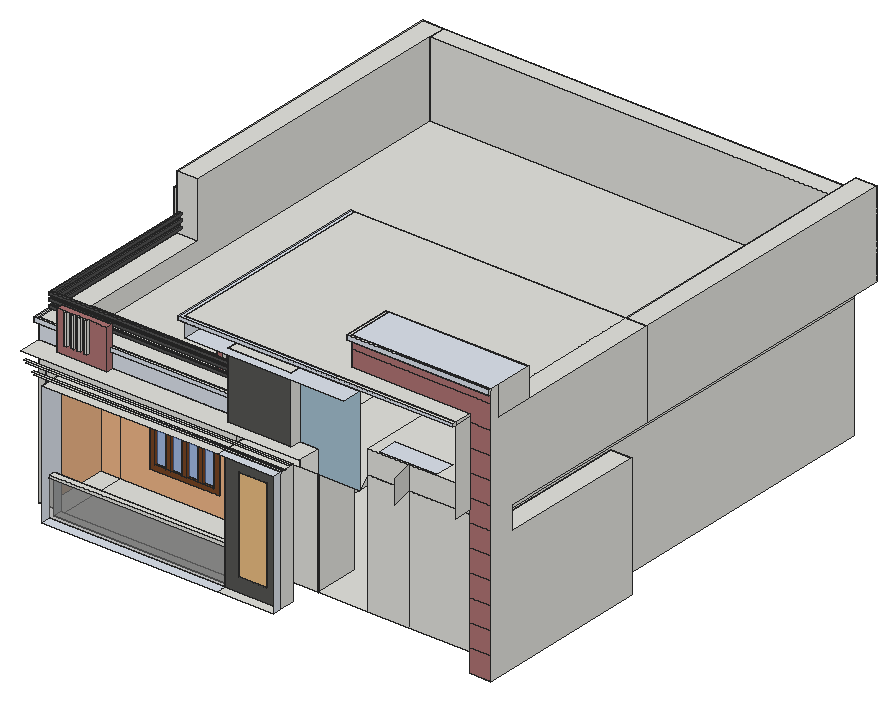
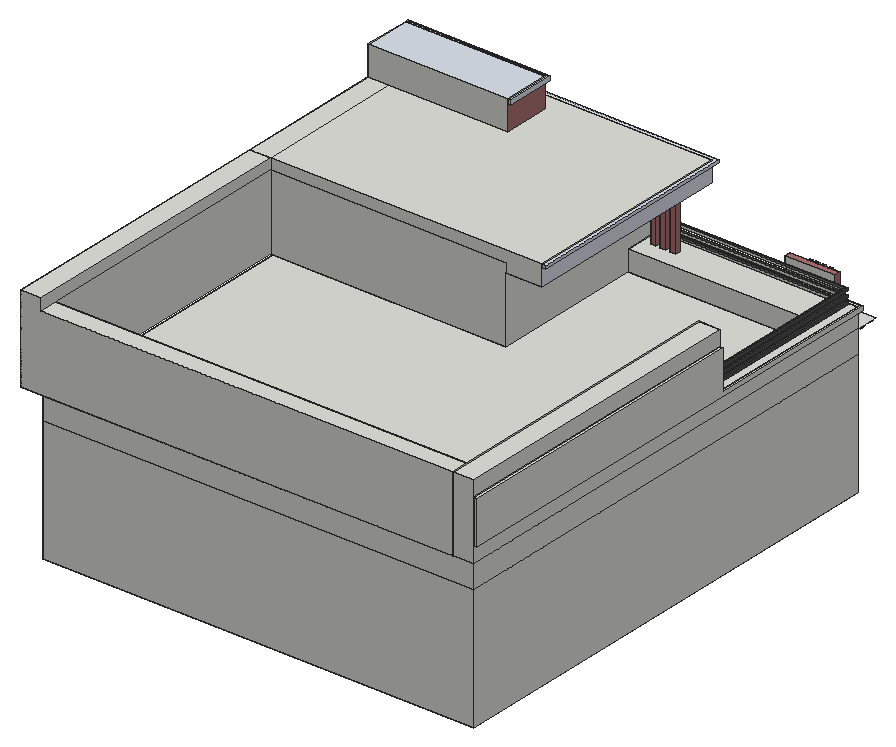
# SketchUp Ruby script. Lengths in inches.
U = 1.inch
M = Sketchup.active_model
def pt(a) = Geom::Point3d.new(a.map { |v| v * U })
def face(e, loops, mat)
  f = e.add_face(loops[0].map { |a| pt(a) })
  loops[1..].each { |l| e.add_face(l.map { |a| pt(a) }).erase! }
  f.material = f.back_material = mat if mat
  f
end
# faces: each face lists its corners as indices into pts; further lists are holes
def faces(e, pts, list, mat = nil) = list.each { |f| face(e, (f[0].is_a?(Array) ? f : [f]).map { |l| l.map { |i| pts[i] } }, mat) }
# xy, xz, yz: faces in a plane at the given z, y or x. An outline is a flat list of corners, or four numbers for a rectangle; further outlines are holes
def ring(l) = l.size == 4 ? [[l[0], l[1]], [l[2], l[1]], [l[2], l[3]], [l[0], l[3]]] : l.each_slice(2).to_a
def flat(e, list, mat, &to3) = list.each { |f| face(e, (f[0].is_a?(Array) ? f : [f]).map { |l| ring(l).map { |u, v| to3.(u, v) } }, mat) }
def xy(e, z, list, mat = nil) = flat(e, list, mat) { |x, y| [x, y, z] }
def xz(e, y, list, mat = nil) = flat(e, list, mat) { |x, z| [x, y, z] }
def yz(e, x, list, mat = nil) = flat(e, list, mat) { |y, z| [x, y, z] }
def lines(e, pts, list) = list.each { |a, b| e.add_line(pt(pts[a]), pt(pts[b])) }
# prism: a flat outline (further loops are holes) pulled along v
def prism(e, loops, v, mat = nil)
  f = face(e, loops, mat); d = Geom::Vector3d.new(v.map { |x| x * U })
  f.pushpull(f.normal.samedirection?(d) ? d.length : -d.length)
end
def box(e, o, s, mat = nil) = prism(e, [[o, [o[0] + s[0], o[1], o[2]], [o[0] + s[0], o[1] + s[1], o[2]], [o[0], o[1] + s[1], o[2]]]], [0, 0, s[2]], mat)
def at(x, y, z, deg = 0) = Geom::Transformation.translation(pt([x, y, z])) * Geom::Transformation.rotation(ORIGIN, Z_AXIS, deg.degrees)
def axes(o, x, y, z) = Geom::Transformation.new([*x, 0, *y, 0, *z, 0, *pt(o).to_a, 1])
def part(name) = M.definitions.add(name)
# library, detail: a bought-in or finely detailed component or shape, given as its bounding box
def library(name, o, s) = part(name).tap { |d| box(d.entities, o, s) }
def detail(e, o, s) = box(e.add_group.entities, o, s)
def put(e, d, t, mat = nil) = e.add_instance(d, t).tap { |i| i.material = mat if mat }
def group(e, t, mat = nil) = e.add_group.tap { |g| g.transformation = t; g.material = mat if mat }.entities
root = M.entities
M.materials.add("Generic").color = [175, 116, 116]
M.materials.add("Generic\#2").color = [164, 192, 208]
M.materials.add("Generic\#3").color = [219, 225, 235]
M.materials.add("Generic\#4").color = [240, 183, 136]
M.materials.add("[0135_DarkGray]").color = [81, 81, 81]
M.materials.add("[Granite Light Gray]").color = [86, 86, 83]
M.materials.add("[Translucent Glass Blue]").color = [100, 149, 237]
M.materials["[Translucent Glass Blue]"].alpha = 0.5
M.materials.add("[Translucent Glass Gray]").color = [128, 128, 128]
M.materials["[Translucent Glass Gray]"].alpha = 0.5
M.materials.add("[Wood Veneer 01]").color = [120, 70, 37]
c1 = library("Group\#6",[0,0,0],[40.87,87.01,0.59])
xy(root,142.6875,[[195.4375,77.59,250.5625,86.22],[195.4375,86.22,250.5625,100.72],[195.4375,91.75,195.4375,100.72,24.3125,100.72,24.3125,91.92],[425.125,98.72,445.5,270.09],[3.0625,100.72,3.0625,568.65,423.0625,568.65,423.0625,175.9,304.375,175.9,304.375,124.65,256.02,124.65,256.02,168.65,9.0625,168.65,9.0625,100.72],
  [9.0625,100.72,28.3125,168.65],[28.3125,100.72,28.3125,168.65,256.02,168.65,256.02,124.65,195.4375,124.65,195.4375,100.72],[304.375,124.65,423.0625,175.9]])
xy(root,142.6875,[[24.3125,77.59,195.4375,77.59,195.4375,86.22,24.3125,86.39]],"Generic\#3")
xy(root,148.78,[[149.02,168.65,188.52,344.59]])
xy(root,156.78,[[209.53,86.22,236.47,90.65]])
xy(root,160.95,[[56.18,168.65,124.43,344.59]])
xy(root,178,[[195.4375,86.22,24.3125,86.39,24.3125,91.92,195.4375,91.75]])
xy(root,181,[[195.4375,86.22,195.4375,91.75,24.3125,91.92,24.3125,86.39]])
xy(root,227.7,[[56.18,168.65,124.43,344.59]])
xy(root,229.03,[[149.02,168.65,188.52,344.59]])
xy(root,248.59,[[209.53,86.22,236.47,90.65]])
xy(root,262.6875,[[24.3125,77.59,195.4375,100.72],[195.4375,86.22,195.4375,124.65,257,124.65,257,100.72,250.5625,100.72,250.5625,86.22],[3.0625,100.72,3.0625,568.65,423.0625,568.65,423.0625,175.9,304.375,175.9,304.375,124.65,316,100.72,257,100.72,257,124.65,256.02,124.65,256.02,168.65,9.0625,168.65,9.0625,100.72],[9.0625,100.72,28.3125,168.65],[28.3125,100.72,28.3125,168.65,256.02,168.65,256.02,124.65,195.4375,124.65,195.4375,100.72],
  [304.375,124.65,423.0625,175.9],[425.125,124.65,445.5,270.09]])
xy(root,262.6875,[[195.4375,77.59,250.5625,86.22]],"Generic\#3")
xy(root,270.625,[[17.8125,75.97,259.625,77.59]])
xy(root,272.67,[[15.77,75.97,261.67,77.59]])
xy(root,278.3,[[10.13,75.97,267.3,77.59]])
xy(root,280.38,[[8.06,75.97,269.38,77.59]])
xy(root,285.375,[[[3.0625,77.59,274.375,77.59,274.375,100.72,257,100.72,257,90.65,195.4375,90.65,195.4375,100.72,3.0625,100.72],[25.83,93.51,74.7,99.88]],[195.4375,90.65,257,100.72],[3.0625,100.72,3.0625,568.65,23.25,568.65,23.25,139.72,195.4375,139.72,195.4375,100.72],[195.4375,100.72,257,124.65],[423.0625,100.72,425.125,124.65],
  [195.4375,124.65,257,289.03],[304.375,124.65,423.0625,289.03],[423.0625,124.65,425.125,289.03],[425.125,124.65,445.5,289.03],[23.25,139.72,195.4375,139.72,195.4375,289.03,423.0625,289.03,423.0625,551.28,23.25,551.28],
  [425.125,289.03,425.125,551.28,423.0625,551.28,423.0625,568.65,445.5,568.65,445.5,289.03],[23.25,551.28,423.0625,568.65]])
xy(root,294.7,[[34.08,91.94,37.39,93.51],[40.58,91.94,43.89,93.51],[47.08,91.94,50.39,93.51],[53.58,91.94,56.89,93.51]])
xy(root,301.3125,[[0,97.65,0,568.65,3.0625,568.65,3.0625,100.72,195.4375,100.72,195.4375,97.65]])
xy(root,305.0625,[[0,97.65,195.4375,97.65,195.4375,100.72,3.0625,100.72,3.0625,268.56,0,268.56],[[3.0625,100.72,195.4375,100.72,195.4375,139.72,23.25,139.72,23.25,268.56,3.0625,268.56],[161.83,118.97,167.81,123.29],[171.57,118.97,177.49,123.29],[181.31,118.97,186.72,123.29]]])
xy(root,317.5625,[[350.4375,81.53,406.3,100.72]],"Generic\#3")
xy(root,324.14,[[34.08,91.94,37.39,93.51],[40.58,91.94,43.89,93.51],[47.08,91.94,50.39,93.51],[53.58,91.94,56.89,93.51]])
xy(root,324.14,[[25.83,93.51,74.7,99.88]],"Generic")
xy(root,343.9375,[[0,268.56,3.0625,568.65]])
xy(root,349.9375,[[195.4375,90.65,257,100.72],[160.125,100.72,195.4375,289.03]])
xy(root,349.9375,[[160.125,81.53,160.125,100.72,195.4375,100.72,195.4375,90.65,257,90.65,257,100.72,316,100.72,316,81.53]],"Generic\#3")
xy(root,355.6875,[[161.83,118.97,167.81,123.29],[171.57,118.97,177.49,123.29],[181.31,118.97,186.72,123.29]])
xy(root,358.8125,[[3.0625,268.56,23.25,568.65],[23.25,551.28,425.125,568.65]])
xy(root,366.8125,[[156.8125,77.97,156.8125,289.03,160.125,289.03,160.125,81.53,193.5,81.53,193.5,77.97],[193.5,77.97,425.125,81.53]])
xy(root,369.6875,[[309.3125,77.97,425.125,81.53],[160.125,81.53,425.125,81.53,425.125,98.72,309.3125,98.72,309.3125,144.28,425.125,144.28,425.125,289.03,160.125,289.03],[425.125,144.28,445.5,289.03],[425.125,289.03,445.5,568.65]])
xy(root,369.6875,[[156.8125,77.97,309.3125,77.97,309.3125,81.53,160.125,81.53,160.125,289.03,156.8125,289.03]],"Generic\#3")
xy(root,393.625,[[306.625,96.53,306.625,144.28,309.3125,144.28,309.3125,98.72,445.5,98.72,445.5,96.53]])
xy(root,398.0625,[[306.625,96.53,445.5,96.53,445.5,98.72,309.3125,98.72,309.3125,144.28,306.625,144.28]])
xy(root,398.0625,[[309.3125,98.72,445.5,144.28]],"Generic\#3")
xz(root,77.97,[[156.8125,366.8125,425.125,369.6875]],"Generic\#3")
xz(root,81.53,[[160.125,366.8125,193.5,369.6875],[193.5,366.8125,425.125,369.6875]])
xz(root,86.22,[[[195.4375,142.6875,250.5625,262.6875],[209.53,156.78,236.47,248.59]]],"[Granite Light Gray]")
xz(root,90.65,[[209.53,156.78,236.47,248.59]])
xz(root,90.65,[[195.4375,285.375,257,349.9375]],"[Granite Light Gray]")
xz(root,91.94,[[34.08,294.7,37.39,324.14],[40.58,294.7,43.89,324.14],[47.08,294.7,50.39,324.14],[53.58,294.7,56.89,324.14]])
xz(root,93.51,[[34.08,294.7,37.39,324.14],[40.58,294.7,43.89,324.14],[47.08,294.7,50.39,324.14],[53.58,294.7,56.89,324.14]])
xz(root,93.51,[[25.83,285.375,74.7,285.375,74.7,324.14,56.89,324.14,56.89,294.7,53.58,294.7,53.58,324.14,50.39,324.14,50.39,294.7,47.08,294.7,47.08,324.14,43.89,324.14,43.89,294.7,40.58,294.7,40.58,324.14,37.39,324.14,37.39,294.7,34.08,294.7,34.08,324.14,25.83,324.14]],"Generic")
xz(root,96.53,[[306.625,393.625,445.5,398.0625]],"Generic\#3")
xz(root,97.65,[[0,301.3125,195.4375,305.0625]],"Generic\#3")
xz(root,98.72,[[309.3125,393.625,445.5,398.0625]])
xz(root,98.72,[[425.125,142.6875,445.5,164.62],[425.125,164.62,445.5,186.55],[425.125,186.55,445.5,208.48],[425.125,208.48,445.5,230.41],[425.125,230.41,445.5,252.35],
  [425.125,252.35,445.5,274.28],[425.125,274.28,445.5,296.21],[425.125,296.21,445.5,318.14],[425.125,318.14,445.5,340.07],[425.125,340.07,445.5,362],
  [425.125,362,445.5,362,445.5,385.625,309.3125,385.625,309.3125,369.6875,425.125,369.6875],[309.3125,385.625,445.5,393.625]],"Generic")
xz(root,99.88,[[25.83,285.375,74.7,324.14]])
xz(root,100.72,[[9.0625,142.6875,24.3125,262.6875],[3.0625,262.6875,195.4375,285.375],[257,262.6875,274.375,285.375],[423.0625,262.6875,425.125,285.375],[195.4375,285.375,257,349.9375],
  [3.0625,301.3125,195.4375,305.0625]])
xz(root,100.72,[[274.375,262.6875,316,262.6875,316,349.9375,257,349.9375,257,285.375,274.375,285.375]],"Generic\#2")
xz(root,100.72,[[3.0625,285.375,195.4375,301.3125]],"Generic\#3")
xz(root,118.97,[[161.83,305.0625,167.81,355.6875],[171.57,305.0625,177.49,355.6875],[181.31,305.0625,186.72,355.6875]],"Generic")
xz(root,123.29,[[161.83,305.0625,167.81,355.6875],[171.57,305.0625,177.49,355.6875],[181.31,305.0625,186.72,355.6875]],"Generic")
xz(root,124.65,[[195.4375,142.6875,256.02,262.6875],[256.02,142.6875,257,262.6875],[304.375,142.6875,344.25,262.6875],[344.25,142.6875,423.0625,262.6875],[195.4375,262.6875,257,285.375],
  [304.375,262.6875,344.25,285.375],[344.25,262.6875,425.125,285.375],[425.125,262.6875,445.5,285.375]])
xz(root,139.72,[[23.25,285.375,195.4375,305.0625]])
xz(root,144.28,[[309.3125,369.6875,445.5,398.0625],[306.625,393.625,309.3125,398.0625]])
xz(root,168.65,[[9.0625,142.6875,28.3125,262.6875],[[28.3125,142.6875,256.02,262.6875],[56.18,160.95,124.43,227.7],[149.02,148.78,188.52,229.03]]],"Generic\#4")
xz(root,175.9,[[304.375,142.6875,423.0625,262.6875]])
xz(root,268.56,[[0,305.0625,3.0625,343.9375],[3.0625,305.0625,23.25,358.8125]])
xz(root,270.09,[[425.125,142.6875,445.5,262.6875]])
xz(root,270.23,[[7.9,321.65,5.61,321.7,5.59,324.14,7.875,324.09]])
xz(root,271.04,[[7.9,316.02,5.61,316.07,5.59,318.52,7.875,318.47]])
xz(root,273.16,[[7.9,309.96,5.61,310.01,5.59,312.46,7.875,312.4]])
xz(root,289.03,[[195.4375,285.375,195.4375,358.5625,257,358.5625,257,358.8125,425.125,358.8125,425.125,285.375],[425.125,285.375,445.5,369.6875],[160.125,349.9375,160.125,369.6875,425.125,369.6875,425.125,358.8125,257,358.8125,257,358.5625,195.4375,358.5625,195.4375,349.9375],[156.8125,366.8125,160.125,369.6875]])
xz(root,344.59,[[149.02,148.78,188.52,229.03],[56.18,160.95,124.43,227.7]])
xz(root,551.28,[[23.25,285.375,425.125,358.8125]])
xz(root,568.65,[[3.0625,142.6875,423.0625,262.6875],[3.0625,262.6875,423.0625,285.375],[3.0625,285.375,23.25,358.8125],[23.25,285.375,23.25,358.8125,425.125,358.8125,425.125,369.6875,445.5,369.6875,445.5,285.375],[0,301.3125,3.0625,343.9375]])
yz(root,0,[[97.65,301.3125,97.65,305.0625,268.56,305.0625,268.56,343.9375,568.65,343.9375,568.65,301.3125]])
yz(root,3.0625,[[100.72,142.6875,568.65,262.6875],[100.72,262.6875,568.65,285.375],[100.72,285.375,568.65,301.3125],[100.72,301.3125,568.65,301.3125,568.65,343.9375,268.56,343.9375,268.56,305.0625,100.72,305.0625],[268.56,343.9375,568.65,358.8125]])
yz(root,9.0625,[[100.72,142.6875,168.65,262.6875]],"Generic\#4")
yz(root,23.25,[[139.72,285.375,551.28,285.375,551.28,358.8125,268.56,358.8125,268.56,305.0625,139.72,305.0625],[551.28,285.375,568.65,358.8125]])
yz(root,24.3125,[[86.39,178,91.92,181]])
yz(root,24.3125,[[77.59,142.6875,86.39,142.6875,86.39,181,91.92,181,91.92,142.6875,100.72,142.6875,100.72,262.6875,77.59,262.6875]],"Generic\#3")
yz(root,25.83,[[93.51,285.375,99.88,324.14]],"Generic")
yz(root,34.08,[[91.94,294.7,93.51,324.14]])
yz(root,37.39,[[91.94,294.7,93.51,324.14]])
yz(root,40.58,[[91.94,294.7,93.51,324.14]])
yz(root,43.89,[[91.94,294.7,93.51,324.14]])
yz(root,47.08,[[91.94,294.7,93.51,324.14]])
yz(root,50.39,[[91.94,294.7,93.51,324.14]])
yz(root,53.58,[[91.94,294.7,93.51,324.14]])
yz(root,56.18,[[168.65,160.95,344.59,227.7]])
yz(root,56.89,[[91.94,294.7,93.51,324.14]])
yz(root,74.7,[[93.51,285.375,99.88,324.14]],"Generic")
yz(root,124.43,[[168.65,160.95,344.59,227.7]])
yz(root,149.02,[[168.65,148.78,344.59,229.03]])
yz(root,156.8125,[[77.97,366.8125,289.03,369.6875]],"Generic\#3")
yz(root,160.125,[[81.53,366.8125,289.03,369.6875]])
yz(root,160.125,[[81.53,349.9375,289.03,366.8125]],"Generic\#3")
yz(root,161.83,[[118.97,305.0625,123.29,355.6875]],"Generic")
yz(root,167.81,[[118.97,305.0625,123.29,355.6875]])
yz(root,171.57,[[118.97,305.0625,123.29,355.6875]],"Generic")
yz(root,177.49,[[118.97,305.0625,123.29,355.6875]])
yz(root,181.31,[[118.97,305.0625,123.29,355.6875]],"Generic")
yz(root,186.72,[[118.97,305.0625,123.29,355.6875]])
yz(root,188.52,[[168.65,148.78,344.59,229.03]])
yz(root,195.4375,[[86.22,142.6875,91.75,178],[91.75,142.6875,91.75,181,86.22,181,86.22,262.6875,124.65,262.6875,124.65,142.6875],[86.22,178,91.75,181],[100.72,262.6875,124.65,285.375],[90.65,285.375,90.65,349.9375,100.72,349.9375,100.72,305.0625,97.65,305.0625,97.65,301.3125,100.72,301.3125,100.72,285.375],
  [100.72,285.375,124.65,305.0625],[[139.72,285.375,139.72,305.0625,100.72,305.0625,100.72,349.9375,289.03,349.9375,289.03,285.375],[111.875,321.65,111.85,324.09,109.5625,324.14,109.59,321.7],[111.875,316.02,111.85,318.47,109.5625,318.52,109.59,316.07],[111.875,309.96,111.85,312.4,109.5625,312.46,109.59,310.01]],[124.65,285.375,139.72,305.0625],[97.65,301.3125,100.72,305.0625],[111.875,309.96,111.85,312.4,109.5625,312.46,109.59,310.01],
  [111.875,316.02,111.85,318.47,109.5625,318.52,109.59,316.07],[111.875,321.65,111.85,324.09,109.5625,324.14,109.59,321.7]])
yz(root,209.53,[[86.22,156.78,90.65,248.59]])
yz(root,236.47,[[86.22,156.78,90.65,248.59]])
yz(root,250.5625,[[86.22,142.6875,100.72,262.6875]])
yz(root,250.5625,[[77.59,142.6875,86.22,262.6875]],"Generic\#3")
yz(root,256.02,[[124.65,142.6875,168.65,262.6875]])
yz(root,257,[[100.72,262.6875,124.65,285.375],[90.65,285.375,100.72,349.9375],[100.72,358.5625,289.03,358.8125]])
yz(root,306.625,[[96.53,393.625,144.28,398.0625]],"Generic\#3")
yz(root,309.3125,[[98.72,393.625,144.28,398.0625]])
yz(root,309.3125,[[98.72,369.6875,144.28,393.625]],"Generic")
yz(root,423.0625,[[175.9,142.6875,568.65,262.6875],[100.72,262.6875,568.65,285.375]])
yz(root,425.125,[[100.72,142.6875,100.72,285.375,124.65,285.375,124.65,262.6875,270.09,262.6875,270.09,142.6875],[81.53,285.375,98.72,366.8125],[289.03,285.375,551.28,358.8125],[289.03,358.8125,568.65,369.6875],[77.97,366.8125,81.53,369.6875],
  [81.53,366.8125,98.72,369.6875]])
yz(root,445.5,[[98.72,142.6875,270.09,142.6875,270.09,262.6875,124.65,262.6875,124.65,285.375,289.03,285.375,289.03,369.6875,106.72,369.6875,106.72,398.0625,98.72,398.0625],[289.03,285.375,568.65,369.6875],[106.72,369.6875,144.28,398.0625],[96.53,393.625,98.72,398.0625]])
p = [[24.3125,86.39,142.6875],[195.4375,86.22,142.6875],[195.4375,86.22,178],[24.3125,86.39,178],[195.4375,91.75,142.6875],[24.3125,91.92,142.6875],
  [24.3125,91.92,178],[195.4375,91.75,178],[195.4375,86.22,181],[24.3125,86.39,181],[24.3125,91.92,181],[195.4375,91.75,181],
  [344.25,124.65,262.6875],[344.25,124.65,285.375],[350.4375,100.72,285.375],[350.4375,100.72,262.6875],[195.4375,111.875,309.96],[195.4375,109.59,310.01],
  [5.61,109.59,310.01],[7.9,111.875,309.96],[5.61,273.16,310.01],[7.9,273.16,309.96],[195.4375,109.5625,312.46],[5.59,109.5625,312.46],
  [5.59,273.16,312.46],[195.4375,111.85,312.4],[7.875,111.85,312.4],[7.875,273.16,312.4],[195.4375,111.875,316.02],[195.4375,109.59,316.07],
  [5.61,109.59,316.07],[7.9,111.875,316.02],[5.61,271.04,316.07],[7.9,271.04,316.02],[195.4375,111.85,318.47],[7.875,111.85,318.47],
  [7.875,271.04,318.47],[195.4375,109.5625,318.52],[5.59,109.5625,318.52],[5.59,271.04,318.52],[195.4375,111.875,321.65],[195.4375,109.59,321.7],
  [5.61,109.59,321.7],[7.9,111.875,321.65],[5.61,270.23,321.7],[7.9,270.23,321.65],[195.4375,111.85,324.09],[7.875,111.85,324.09],
  [7.875,270.23,324.09],[195.4375,109.5625,324.14],[5.59,109.5625,324.14],[5.59,270.23,324.14],[304.375,289.03,358.8125],[304.375,100.72,358.8125],
  [304.375,100.72,358.5625],[257,100.72,358.5625],[257,100.72,349.9375],[195.4375,110.54,311.17],[6.5625,110.54,311.17],[6.5625,257.35,311.17],
  [6.5625,110.54,317.04],[6.5625,257.35,317.04],[195.4375,110.54,317.04],[6.5625,110.54,322.92],[6.5625,257.35,322.92],[195.4375,110.54,322.92]]
faces(root,p,[[0,1,2,3],[4,5,6,7]],"[Translucent Glass Gray]")
faces(root,p,[[3,2,8,9],[7,6,10,11],[12,13,14,15],[16,17,18,19],[19,18,20,21],[25,16,19,26],[28,29,30,31],[31,30,32,33],
  [34,28,31,35],[40,41,42,43],[43,42,44,45],[46,40,43,47]])
faces(root,p,[[17,22,23,18],[18,23,24,20],[26,19,21,27],[22,25,26,23],[23,26,27,24],[35,31,33,36],[29,37,38,30],[30,38,39,32],
  [37,34,35,38],[38,35,36,39],[47,43,45,48],[41,49,50,42],[42,50,51,44],[49,46,47,50],[50,47,48,51]],"[0135_DarkGray]")
lines(root,p,[[52,53],[54,53],[55,56],[57,58],[58,59],[60,61],[62,60],[63,64],[65,63]])
g1 = group(root,at(149.02,168.65,148.78))
p = [[5.01,0.77,38.29],[8.11,3.52,33.37],[5.01,3.52,38.29]]
lines(g1,p,[[0,1],[2,0]])
detail(g1,[0,0,0],[39.5,7.14,80.25])
put(root,c1,axes([209.53,86.81,156.97],[0.65906,0,0],[0,0,1.05307],[0,-1,0]))
g2 = group(root,at(56.18,168.65,160.95))
xy(g2,0,[[0,0,68.25,3.8125]])
xy(g2,4.94,[[4.94,0,15.83,2.375],[20.77,0,31.65,2.375],[36.6,0,47.48,2.375],[52.42,0,63.31,2.375]],"[Wood Veneer 01]")
xy(g2,61.81,[[4.94,0,15.83,2.375],[20.77,0,31.65,2.375],[36.6,0,47.48,2.375],[52.42,0,63.31,2.375]])
xy(g2,66.75,[[0,0,68.25,3.8125]],"[Wood Veneer 01]")
xz(g2,0,[[[0,0,68.25,66.75],[4.94,4.94,63.31,61.81]],[15.83,4.94,20.77,61.81],[31.65,4.94,36.6,61.81],[47.48,4.94,52.42,61.81]],"[Wood Veneer 01]")
xz(g2,2.375,[[4.94,4.94,15.83,61.81],[20.77,4.94,31.65,61.81],[36.6,4.94,47.48,61.81],[52.42,4.94,63.31,61.81]],"[Translucent Glass Blue]")
xz(g2,3.8125,[[0,0,68.25,66.75]])
yz(g2,0,[[0,0,3.8125,66.75]],"[Wood Veneer 01]")
yz(g2,4.94,[[0,4.94,2.375,61.81]],"[Wood Veneer 01]")
yz(g2,15.83,[[0,4.94,2.375,61.81]],"[Wood Veneer 01]")
yz(g2,20.77,[[0,4.94,2.375,61.81]],"[Wood Veneer 01]")
yz(g2,31.65,[[0,4.94,2.375,61.81]],"[Wood Veneer 01]")
yz(g2,36.6,[[0,4.94,2.375,61.81]],"[Wood Veneer 01]")
yz(g2,47.48,[[0,4.94,2.375,61.81]],"[Wood Veneer 01]")
yz(g2,52.42,[[0,4.94,2.375,61.81]],"[Wood Veneer 01]")
yz(g2,63.31,[[0,4.94,2.375,61.81]],"[Wood Veneer 01]")
yz(g2,68.25,[[0,0,3.8125,66.75]],"[Wood Veneer 01]")
